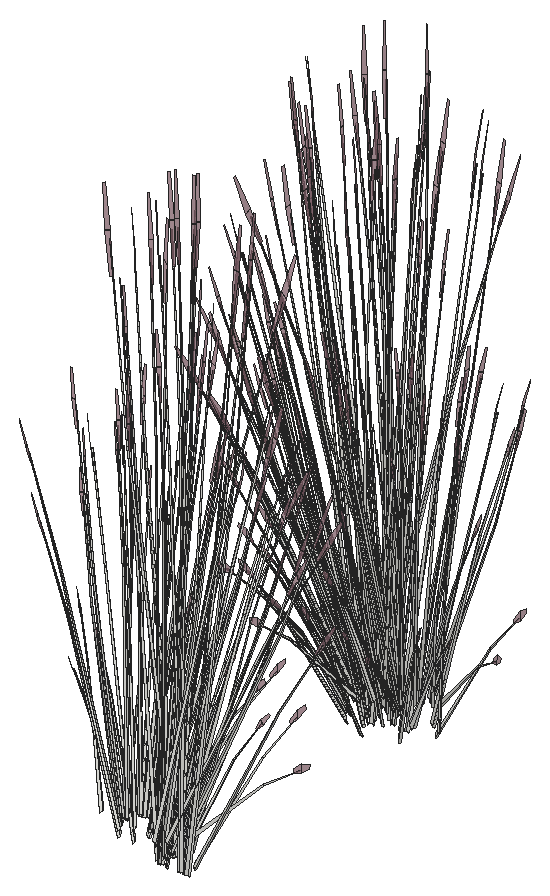
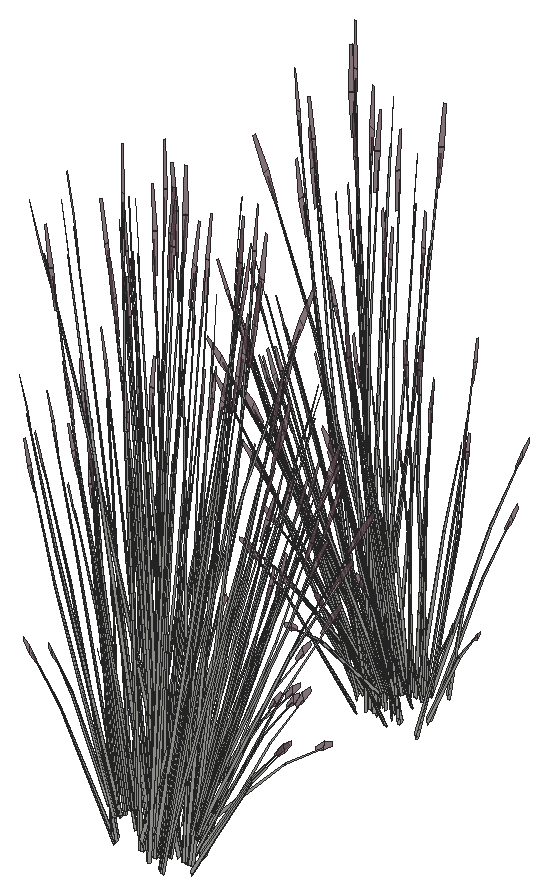
# SketchUp Ruby script. Lengths in inches.
U = 1.inch
M = Sketchup.active_model
def pt(a) = Geom::Point3d.new(a.map { |v| v * U })
def face(e, loops, mat)
  f = e.add_face(loops[0].map { |a| pt(a) })
  loops[1..].each { |l| e.add_face(l.map { |a| pt(a) }).erase! }
  f.material = f.back_material = mat if mat
  f
end
# faces: each face lists its corners as indices into pts; further lists are holes
def faces(e, pts, list, mat = nil) = list.each { |f| face(e, (f[0].is_a?(Array) ? f : [f]).map { |l| l.map { |i| pts[i] } }, mat) }
# xy, xz, yz: faces in a plane at the given z, y or x. An outline is a flat list of corners, or four numbers for a rectangle; further outlines are holes
def ring(l) = l.size == 4 ? [[l[0], l[1]], [l[2], l[1]], [l[2], l[3]], [l[0], l[3]]] : l.each_slice(2).to_a
def flat(e, list, mat, &to3) = list.each { |f| face(e, (f[0].is_a?(Array) ? f : [f]).map { |l| ring(l).map { |u, v| to3.(u, v) } }, mat) }
def xy(e, z, list, mat = nil) = flat(e, list, mat) { |x, y| [x, y, z] }
def xz(e, y, list, mat = nil) = flat(e, list, mat) { |x, z| [x, y, z] }
def yz(e, x, list, mat = nil) = flat(e, list, mat) { |y, z| [x, y, z] }
def lines(e, pts, list) = list.each { |a, b| e.add_line(pt(pts[a]), pt(pts[b])) }
# prism: a flat outline (further loops are holes) pulled along v
def prism(e, loops, v, mat = nil)
  f = face(e, loops, mat); d = Geom::Vector3d.new(v.map { |x| x * U })
  f.pushpull(f.normal.samedirection?(d) ? d.length : -d.length)
end
def box(e, o, s, mat = nil) = prism(e, [[o, [o[0] + s[0], o[1], o[2]], [o[0] + s[0], o[1] + s[1], o[2]], [o[0], o[1] + s[1], o[2]]]], [0, 0, s[2]], mat)
def at(x, y, z, deg = 0) = Geom::Transformation.translation(pt([x, y, z])) * Geom::Transformation.rotation(ORIGIN, Z_AXIS, deg.degrees)
def axes(o, x, y, z) = Geom::Transformation.new([*x, 0, *y, 0, *z, 0, *pt(o).to_a, 1])
def part(name) = M.definitions.add(name)
# library, detail: a bought-in or finely detailed component or shape, given as its bounding box
def library(name, o, s) = part(name).tap { |d| box(d.entities, o, s) }
def detail(e, o, s) = box(e.add_group.entities, o, s)
def put(e, d, t, mat = nil) = e.add_instance(d, t).tap { |i| i.material = mat if mat }
def group(e, t, mat = nil) = e.add_group.tap { |g| g.transformation = t; g.material = mat if mat }.entities
root = M.entities
M.materials.add("LightPink_Translucent").color = [144, 107, 117]
M.materials["LightPink_Translucent"].alpha = 0.75
c1 = part("blade")
p = [[2.15,0.21,22],[0,0.17,0],[0.09,0.45,0],[2.18,0.31,22],[2.29,0.31,22],[0.38,0.45,0],
  [2.48,0.24,33],[2.49,0.24,33],[2.48,0.22,33]]
faces(c1.entities,p,[[0,1,2,3],[4,5,2,3],[6,3,4,7],[8,0,3,6]])
c2 = part("seeds")
p = [[0.3,-0.1,1.38],[-0.01,-0.03,1.59],[-0.01,-0.03,0.03],[0.14,-0.07,-0.07],[0.29,-0.03,3],[0.15,0.01,3.11]]
faces(c2.entities,p,[[0,1,2,3],[1,0,4,5]],"LightPink_Translucent")
c3 = part("blade with seeds")
put(c3.entities,c1,at(0,0,0))
put(c3.entities,c2,axes([2.4,0.25,30.99],[1.5799,-0.05474,1.17369],[-0.12525,1.92788,0.29478],[-0.07173,-0.02425,1.56792]))
put(root,c3,axes([360.53,227.94,49.94],[-0.13408,-0.12117,1.07251],[0.17446,-0.40083,-0.23066],[0.27128,0.0543,0.45856]))
put(root,c3,axes([358.14,228.38,49.65],[0.56127,0.22118,0],[-0.27012,0.45959,0],[0,0,1.31215]))
put(root,c3,axes([359.76,228.125,51.54],[0.11943,-0.00833,1.31208],[0.32759,-0.38275,-0.2075],[0.21244,0.05052,0.10523]))
put(root,c3,axes([358.36,228.87,49.64],[-0.34375,-0.4954,-0.03857],[0.58235,-0.27531,0.38706],[-0.1435,0.04717,1.22723]))
put(root,c3,axes([358.24,227.67,49.96],[0.41131,0.296,0.1086],[-0.34309,0.33395,-0.3101],[-0.0955,0.04515,0.95058]))
put(root,c3,axes([354.99,227.75,51.55],[-0.13808,-0.45342,0.36002],[0.54163,-0.07869,0.29685],[-0.15963,0.10664,0.74497]))
put(root,c3,axes([354.88,227.66,51.55],[-0.3822,-0.20719,0.04823],[0.22252,-0.29505,0.37966],[-0.12254,0.09539,0.57892]))
put(root,c3,axes([355.06,227.12,50.91],[0.19317,-0.10421,1.28532],[0.16263,0.48153,0.10393],[-0.30326,0.10883,0.54946]))
put(root,c3,axes([359.3,228.1875,51.74],[0.55654,0.01186,-0.53284],[-0.03738,0.49951,0.0643],[0.23578,0.05271,0.75375]))
put(root,c3,axes([358.67,228.59,49.86],[0.52105,-0.24633,0.37238],[0.31144,0.44171,0],[-0.11867,0.0561,1.18128]))
put(root,c3,axes([357.93,228.2,49.72],[0.24206,0.56598,-0.04509],[-0.69162,0.19832,0],[0.00845,0.01976,1.2913]))
put(root,c3,axes([358.2,228.81,49.52],[-0.51941,-0.1219,-0.23233],[0.13078,-0.42928,0.23233],[-0.10471,0.0495,1.0423]))
put(root,c3,axes([354.45,227.9375,49.94],[0.19348,0.04044,1.07251],[0.1247,0.41309,-0.23066],[-0.26282,0.07733,0.45856]))
put(root,c3,axes([355.32,227.6,51.79],[0.48462,-0.07041,0.2656],[0.12797,0.4025,-0.3429],[-0.13888,0.10811,0.65611]))
put(root,c3,axes([360.21,227.17,49.78],[0.69617,0,0],[0,0.55062,-0.38706],[0,0.12541,1.22783]))
put(root,c3,axes([353.46,227.42,51.53],[0.07105,0.01321,1.33037],[0.2198,0.43529,-0.12571],[-0.14545,0.11425,0.23543]))
put(root,c3,axes([359.93,227.46,49.65],[-0.69582,-0.00394,-0.03732],[0,-0.55062,0.37457],[-0.02187,0.12535,1.18764]))
put(root,c3,axes([358.43,226.98,50],[0.62699,0.23507,-0.21822],[-0.3019,0.49615,-0.37502],[0.0197,0.12182,1.19781]))
put(root,c3,axes([354.05,228.8,50.07],[0.23202,-0.22328,0.86145],[0.09155,0.35348,0.63294],[-0.16768,0.06329,0.18974]))
put(root,c3,axes([359.64,228.39,51.39],[0.31678,0.30846,-0.2656],[-0.36171,0.29199,0.3429],[0.18378,0.04443,0.65611]))
put(root,c3,axes([359.79,227.54,49.52],[-0.38863,0.30738,-0.23233],[-0.38863,-0.30738,0.23233],[0,0.09901,1.0423]))
put(root,c3,axes([358.11,227.57,50],[0.06488,0.56215,-0.21822],[-0.6757,0.03399,-0.37502],[-0.11898,0.07488,1.19781]))
put(root,c3,axes([359.47,228.51,51.55],[-0.02803,0.37463,0.04823],[-0.42332,-0.01027,0.37966],[0.16216,0.0392,0.57892]))
put(root,c3,axes([358.36,227.35,49.66],[-0.27012,0.44393,-0.33554],[-0.56127,-0.21365,0.16149],[0,0.10233,1.07733]))
put(root,c3,axes([354.93,227.84,51.39],[-0.48462,0.07041,-0.2656],[-0.12797,-0.4025,0.3429],[-0.13888,0.10811,0.65611]))
put(root,c3,axes([359.51,228.39,51.55],[-0.41051,0.32462,0.36002],[-0.35404,-0.34474,0.29685],[0.1926,0.05988,0.74497]))
put(root,c3,axes([354.22,228.74,52.23],[0.49129,0.13151,-0.04866],[-0.15113,0.40475,-0.22062],[-0.08035,0.06145,0.72768]))
put(root,c3,axes([357.71,227.99,49.54],[-0.375,0.3703,-0.46765],[-0.46584,-0.33578,-0.12274],[-0.15027,0.09237,1.03225]))
put(root,c3,axes([358.21,228.77,51.79],[-0.08599,-0.39682,0.2656],[0.49155,-0.10478,-0.3429],[0.13203,0.11372,0.65611]))
put(root,c3,axes([358.375,228.62,49.75],[0.697,0.16013,0.23067],[-0.17437,0.57237,-0.27369],[-0.11536,0.07164,1.23664]))
put(root,c3,axes([358.32,229,49.51],[-0.52105,0.24633,-0.37238],[-0.31144,-0.44171,0],[-0.11867,0.0561,1.18128]))
put(root,c3,axes([360.06,227.55,49.51],[0,0.49266,-0.37238],[-0.62289,0,0],[0,0.11221,1.18128]))
put(root,c3,axes([358.5,227.6,50.91],[-0.2068,-0.08488,1.28532],[0.42797,-0.35609,0.10393],[0.26673,0.16064,0.54946]))
put(root,c3,axes([358.54,226.48,51.36],[-0.48108,-0.25598,1.03712],[0.50798,-0.39855,0.44749],[0.15521,0.24018,1.00248]))
put(root,c3,axes([355.07,227.5625,51.78],[0.515,0.27165,-0.0912],[-0.2967,0.3934,-0.50621],[-0.1455,0.13675,0.76918]))
put(root,c3,axes([359.26,228.57,50.07],[-0.31347,-0.14166,0.86145],[0.40476,-0.14393,0.63294],[0.10917,0.12192,0.18974]))
put(root,c3,axes([358.16,228.97,51.78],[0.33176,-0.4217,-0.0912],[0.48044,0.24295,-0.50621],[0.16701,0.11914,0.76918]))
put(root,c3,axes([355.76,227.44,50.91],[0.13906,-0.15138,1.28532],[0.35111,0.40859,0.10393],[-0.24082,0.18608,0.54946]))
put(root,c3,axes([355.33,227.89,51.51],[0.14302,0.44985,-0.38324],[-0.54163,0.07869,-0.29685],[-0.15522,0.12083,0.7333]))
put(root,c3,axes([355.98,228.4,51.79],[0.3767,-0.25939,0.2656],[0.3566,0.29618,-0.3429],[-0.05426,0.15048,0.65611]))
put(root,c3,axes([358.8,228.93,49.78],[0.34808,0.49367,0],[-0.58235,0.27531,-0.38706],[-0.13264,0.0627,1.22783]))
put(root,c3,axes([357.73,229.32,51.53],[0.00165,-0.05965,1.33037],[0.47711,-0.26315,-0.12571],[0.16572,0.09393,0.23543]))
put(root,c3,axes([359.35,229.09,49.12],[0.04056,-0.07113,1.32257],[0.51066,-0.20948,-0.20205],[0.15482,0.10842,0.22528]))
put(root,c3,axes([358.5,226.97,50.13],[-0.01521,-0.46386,1.05954],[0.68831,0.12024,0.44862],[-0.1628,0.25382,1.00012]))
put(root,c3,axes([358.68,227.48,49.57],[0.20414,0.45107,-0.51909],[-0.58805,0.16245,-0.13624],[0.02256,0.15274,1.1458]))
put(root,c3,axes([355.63,228.64,51.55],[-0.45752,-0.02296,0.04823],[0.01254,-0.34663,0.37966],[-0.04787,0.13278,0.57892]))
put(root,c3,axes([354.66,229.03,49.12],[0.07468,0.04922,1.32257],[0.12663,0.45605,-0.20205],[-0.16551,0.09725,0.22528]))
put(root,c3,axes([355.78,228.67,51.55],[-0.39645,-0.33614,0.36002],[0.42102,-0.2899,0.29685],[-0.07313,0.15771,0.74497]))
put(root,c3,axes([358.56,228.76,51.51],[0.54938,-0.11711,-0.38324],[0.0961,0.44351,-0.29685],[0.14756,0.1271,0.7333]))
put(root,c3,axes([357.03,228.83,51.79],[0.16784,-0.37886,0.2656],[0.48968,0.1105,-0.3429],[0.0449,0.15254,0.65611]))
put(root,c3,axes([359.3125,229.21,50],[-0.35702,-0.01545,0.78795],[0.23577,-0.32816,0.43504],[0.14104,0.11659,0.61808]))
put(root,c3,axes([358.29,229.125,51.55],[-0.25304,0.31296,0.04823],[-0.36033,-0.18221,0.37966],[0.11649,0.10034,0.57892]))
put(root,c3,axes([357.69,230.18,52.23],[0.38473,-0.28263,-0.04866],[0.35252,0.30954,-0.22062],[0.02482,0.08771,0.72768]))
put(root,c3,axes([358.39,229.04,51.55],[-0.55374,0.11306,0.36002],[-0.0961,-0.44351,0.29685],[0.13023,0.13071,0.74497]))
put(root,c3,axes([355.66,227.82,50.91],[0.10366,-0.16934,1.28532],[0.43488,0.35044,0.10393],[-0.19618,0.21841,0.54946]))
put(root,c3,axes([358.15,228.42,49.94],[0.00982,-0.16331,1.07251],[0.4695,-0.18242,-0.23066],[0.14493,0.19547,0.45856]))
put(root,c3,axes([356.88,229.17,51.55],[-0.41024,0.16744,0.04823],[-0.2008,-0.30532,0.37966],[0.03962,0.13459,0.57892]))
put(root,c3,axes([355.78,228.77,51.39],[-0.3767,0.25939,-0.2656],[-0.3566,-0.29618,0.3429],[-0.05426,0.15048,0.65611]))
put(root,c3,axes([354.48,228.69,51.54],[-0.01384,0.09749,1.31208],[0.39274,0.33916,-0.2075],[-0.10282,0.16039,0.10523]))
put(root,c3,axes([355.74,228.47,52.05],[0.61188,0.02441,-0.10123],[-0.01672,0.46217,-0.56189],[-0.0425,0.178,0.85379]))
put(root,c3,axes([356.87,228.99,51.78],[0.54481,-0.22937,-0.0912],[0.26773,0.4071,-0.50621],[0.07188,0.17155,0.76918]))
put(root,c3,axes([357.03,229.14,51.8],[-0.54859,-0.1288,0.39962],[0.18759,-0.42344,0.32951],[0.03297,0.16652,0.82692]))
put(root,c3,axes([356.02,229.78,50.07],[-0.01441,-0.29294,0.86145],[0.36003,0.20894,0.63294],[-0.07081,0.13963,0.18974]))
put(root,c3,axes([356.97,229.08,49.12],[0.0901,-0.02681,1.32257],[0.54199,0.14755,-0.20205],[0.01585,0.1663,0.22528]))
put(root,c3,axes([356.15,228.65,51.75],[0.39855,0.33102,-0.4254],[-0.42102,0.2899,-0.32951],[-0.06064,0.16819,0.81396]))
put(root,c3,axes([355.72,229.15,50.12],[0.50577,-0.08724,0.04881],[0.11627,0.35148,-0.64728],[-0.03206,0.17792,0.5802]))
put(root,c3,axes([357.34,228.97,51.51],[0.54728,0.1235,-0.38324],[-0.18759,0.42344,-0.29685],[0.05018,0.17048,0.7333]))
put(root,c3,axes([357.65,228.1,50.91],[-0.12726,-0.15818,1.28532],[0.58807,-0.13317,0.10393],[0.13291,0.24832,0.54946]))
put(root,c3,axes([357.09,229.23,51.39],[-0.16784,0.37886,-0.2656],[-0.48968,-0.1105,0.3429],[0.0449,0.15254,0.65611]))
put(root,c3,axes([356.03,228.5,52],[-0.01449,0.45571,-0.59145],[-0.61002,-0.03061,0.07138],[-0.06438,0.19306,0.83667]))
put(root,c3,axes([354.4375,229.69,51.53],[0.06316,-0.02974,1.33037],[0.52204,0.19785,-0.12571],[-0.01227,0.16473,0.23543]))
put(root,c3,axes([356.61,228.17,50.91],[-0.01363,-0.18909,1.28532],[0.5906,0.12544,0.10393],[-0.03653,0.26947,0.54946]))
put(root,c3,axes([357.14,228.89,51.74],[0.26572,0.40059,-0.53284],[-0.54698,0.22325,0.0643],[0.06214,0.19355,0.75375]))
put(root,c3,axes([355.6,229.52,49.94],[0.17569,-0.07772,1.07251],[0.43377,0.23434,-0.23066],[-0.12911,0.20277,0.45856]))
put(root,c3,axes([356.74,229.9,51.54],[0.07057,0.07933,1.31208],[0.56952,0.03117,-0.2075],[0.05727,0.17496,0.10523]))
put(root,c3,axes([355.83,229.14,50.52],[0.01223,-0.25433,1.15759],[0.55017,0.13434,0.15997],[-0.04767,0.27105,0.54661]))
put(root,c3,axes([356.25,248.83,50.91],[0.12726,0.15818,1.28532],[-0.58807,0.13317,0.10393],[-0.13291,-0.24832,0.54946]))
put(root,c3,axes([357.22,247.78,51.54],[-0.08515,-0.06907,1.31208],[-0.56828,0.04379,-0.2075],[-0.0907,-0.16522,0.10523]))
put(root,c3,axes([358.54,248.6,49.94],[-0.15825,0.09972,1.07251],[-0.47395,-0.17454,-0.23066],[0.08785,-0.21706,0.45856]))
put(root,c3,axes([357.82,248.94,51.74],[-0.26572,-0.40059,-0.53284],[0.54698,-0.22325,0.0643],[-0.06214,-0.19355,0.75375]))
put(root,c3,axes([356.09,248.41,49.94],[-0.03371,0.16116,1.07251],[-0.49286,0.13491,-0.23066],[-0.11521,-0.20831,0.45856]))
put(root,c3,axes([357.36,248.06,49.12],[-0.09338,0.01775,1.32257],[-0.51641,-0.1998,-0.20205],[0.00867,-0.16666,0.22528]))
put(root,c3,axes([358.92,249.34,51.74],[0.01449,-0.45571,-0.53284],[0.61002,0.03061,0.0643],[0.06438,-0.19306,0.75375]))
put(root,c3,axes([359.77,248.625,51.54],[-0.00537,-0.09805,1.31208],[-0.45391,-0.28338,-0.2075],[0.07018,-0.17178,0.10523]))
put(root,c3,axes([357.87,248.6,51.39],[0.16784,-0.37886,-0.2656],[0.48968,0.1105,0.3429],[-0.0449,-0.15254,0.65611]))
put(root,c3,axes([358.24,249.1,50.91],[-0.10366,0.16934,1.28532],[-0.43488,-0.35044,0.10393],[0.19618,-0.21841,0.54946]))
put(root,c3,axes([359.65,248.27,51.53],[-0.05654,0.03763,1.33037],[-0.55396,-0.12696,-0.12571],[-0.02005,-0.16422,0.23543]))
put(root,c3,axes([357.62,248.86,51.51],[-0.54728,-0.1235,-0.38324],[0.18759,-0.42344,-0.29685],[-0.05018,-0.17048,0.7333]))
put(root,c3,axes([357.95,247.8,50.07],[0.07142,0.28728,0.86145],[-0.3962,-0.15911,0.63294],[0.04263,-0.1471,0.18974]))
put(root,c3,axes([358.8,249.18,51.51],[-0.39855,-0.33102,-0.38324],[0.42102,-0.2899,-0.29685],[0.06064,-0.16819,0.7333]))
put(root,c3,axes([356.64,247.55,51.53],[-0.01039,0.05905,1.33037],[-0.51226,0.21431,-0.12571],[-0.15074,-0.10955,0.23543]))
put(root,c3,axes([356.52,248.6,51.82],[0.62019,-0.12663,0.40322],[0.10763,0.49673,0.33247],[-0.14586,-0.1464,0.83437]))
put(root,c3,axes([357.93,248.69,51.55],[0.54859,0.1288,0.36002],[-0.18759,0.42344,0.29685],[-0.03297,-0.16652,0.74497]))
put(root,c3,axes([358.08,248.84,51.78],[-0.54481,0.22937,-0.0912],[-0.26773,-0.4071,-0.50621],[-0.07188,-0.17155,0.76918]))
put(root,c3,axes([359.22,249.36,51.78],[-0.61188,-0.02441,-0.0912],[0.01672,-0.46217,-0.50621],[0.0425,-0.178,0.76918]))
put(root,c3,axes([359.17,249.0625,51.39],[0.3767,-0.25939,-0.2656],[0.3566,0.29618,0.3429],[0.05426,-0.15048,0.65611]))
put(root,c3,axes([355.92,248.15,50.07],[0.29042,0.17147,0.86145],[-0.42295,0.10307,0.63294],[-0.0905,-0.13178,0.18974]))
put(root,c3,axes([358.07,248.66,51.55],[0.41024,-0.16744,0.04823],[0.2008,0.30532,0.37966],[-0.03962,-0.13459,0.57892]))
put(root,c3,axes([356.62,249.06,51.74],[-0.47473,-0.23813,-0.53284],[0.33738,-0.41728,0.0643],[-0.172,-0.14218,0.75375]))
put(root,c3,axes([356.45,248.74,51.39],[-0.08599,-0.39682,-0.2656],[0.49155,-0.10478,0.3429],[-0.13203,-0.11372,0.65611]))
put(root,c3,axes([356.67,248.71,51.55],[0.25304,-0.31296,0.04823],[0.36033,0.18221,0.37966],[-0.11649,-0.10034,0.57892]))
put(root,c3,axes([355.6875,248.67,49.12],[-0.05393,0.0649,1.32257],[-0.545,0.13993,-0.20205],[-0.13166,-0.12729,0.22528]))
put(root,c3,axes([356.59,250.45,49.57],[-0.22864,-0.5052,-0.52377],[0.65862,-0.18195,-0.13747],[-0.02527,-0.17107,1.15612]))
put(root,c3,axes([355.4,249.32,50.91],[0.2068,0.08488,1.28532],[-0.42797,0.35609,0.10393],[-0.26673,-0.16064,0.54946]))
put(root,c3,axes([359.64,248.9,49.12],[-0.08333,-0.03881,1.32257],[-0.21404,-0.4336,-0.20205],[0.14439,-0.11767,0.22528]))
put(root,c3,axes([357.92,249,51.79],[-0.16784,0.37886,0.2656],[-0.48968,-0.1105,-0.3429],[-0.0449,-0.15254,0.65611]))
put(root,c3,axes([356.4,249.07,51.51],[-0.54938,0.11711,-0.38324],[-0.0961,-0.44351,-0.29685],[-0.14756,-0.1271,0.7333]))
put(root,c3,axes([359.17,249.16,51.55],[0.39645,0.33614,0.36002],[-0.42102,0.2899,0.29685],[0.07313,-0.15771,0.74497]))
put(root,c3,axes([356.78,248.67,52.07],[-0.37157,0.4723,-0.10215],[-0.5381,-0.2721,-0.56695],[-0.18705,-0.13344,0.86148]))
put(root,c3,axes([359.32,249.19,51.55],[0.45752,0.02296,0.04823],[-0.01254,0.34663,0.37966],[0.04787,-0.13278,0.57892]))
put(root,c3,axes([358.98,249.43,51.79],[-0.3767,0.25939,0.2656],[-0.3566,-0.29618,-0.3429],[0.05426,-0.15048,0.65611]))
put(root,c3,axes([359.64,250.13,51.74],[0.29081,-0.38873,-0.53284],[0.5096,0.27626,0.0643],[0.17364,-0.14084,0.75375]))
put(root,c3,axes([356.5,249,49.78],[-0.34808,-0.49367,0],[0.58235,-0.27531,-0.38706],[0.13264,-0.0627,1.22783]))
put(root,c3,axes([359.625,249.95,51.51],[-0.14302,-0.44985,-0.38324],[0.54163,-0.07869,-0.29685],[0.15522,-0.12083,0.7333]))
put(root,c3,axes([357.26,248.4,49.6],[-0.38473,0.28263,-0.02919],[-0.35252,-0.30954,-0.13237],[-0.02482,-0.08771,0.43661]))
put(root,c3,axes([355.36,248.54,51.54],[-0.11979,-0.00348,1.31208],[-0.38137,0.34775,-0.2075],[-0.20349,-0.07106,0.10523]))
put(root,c3,axes([359.88,250.27,51.78],[-0.515,-0.27165,-0.0912],[0.2967,-0.3934,-0.50621],[0.1455,-0.13675,0.76918]))
put(root,c3,axes([357.75,251.75,50.49],[0.48111,0.19866,1.13446],[-0.47133,0.42798,0.44862],[-0.21112,-0.25366,0.95105]))
put(root,c3,axes([356.75,249.07,51.79],[0.08599,0.39682,0.2656],[-0.49155,0.10478,-0.3429],[-0.13203,-0.11372,0.65611]))
put(root,c3,axes([355.24,250.38,49.51],[0,-0.49266,-0.37238],[0.62289,0,0],[0,-0.11221,1.18128]))
put(root,c3,axes([356.97,248.92,49.51],[0.52105,-0.24633,-0.37238],[0.31144,0.44171,0],[0.11867,-0.0561,1.18128]))
put(root,c3,axes([360.0625,249.77,49.94],[-0.19889,-0.01459,1.07251],[-0.20376,-0.39145,-0.23066],[0.24434,-0.11074,0.45856]))
put(root,c3,axes([355.27,249.32,51.82],[0.45978,-0.36358,0.40322],[0.39653,0.38611,0.33247],[-0.21571,-0.06707,0.83437]))
put(root,c3,axes([361.15,250.15,51.53],[-0.07272,-0.00374,1.33037],[-0.30197,-0.40092,-0.12571],[0.12127,-0.13182,0.23543]))
put(root,c3,axes([357.59,249.93,49.54],[0.375,-0.3703,-0.46765],[0.46584,0.33578,-0.12274],[0.15027,-0.09237,1.03225]))
put(root,c3,axes([360.29,249.05,50.07],[-0.18544,0.25079,0.86145],[-0.15939,-0.33694,0.63294],[0.15316,-0.08443,0.18974]))
put(root,c3,axes([360.03,249.99,51.39],[0.48462,-0.07041,-0.2656],[0.12797,0.4025,0.3429],[0.13888,-0.10811,0.65611]))
put(root,c3,axes([355.48,249.32,51.55],[0.02803,-0.37463,0.04823],[0.42332,0.01027,0.37966],[-0.16216,-0.0392,0.57892]))
put(root,c3,axes([356.93,250.58,49.66],[0.27012,-0.44393,-0.33554],[0.56127,0.21365,0.16149],[0,-0.10233,1.07733]))
put(root,c3,axes([355.32,249.44,51.39],[-0.31678,-0.30846,-0.2656],[0.36171,-0.29199,0.3429],[-0.18378,-0.04443,0.65611]))
put(root,c3,axes([357.18,250.36,50],[-0.06488,-0.56215,-0.21822],[0.6757,-0.03399,-0.37502],[0.11898,-0.07488,1.19781]))
put(root,c3,axes([355.51,250.39,49.52],[0.38863,-0.30738,-0.23233],[0.38863,0.30738,0.23233],[0,-0.09901,1.0423]))
put(root,c3,axes([355.35,248.92,49.6],[-0.1606,0.40228,-0.02919],[-0.4943,-0.12375,-0.13237],[-0.07505,-0.0658,0.43661]))
put(root,c3,axes([359.63,250.23,51.79],[-0.48462,0.07041,0.2656],[-0.12797,-0.4025,-0.3429],[0.13888,-0.10811,0.65611]))
put(root,c3,axes([356.87,250.95,50],[-0.62699,-0.23507,-0.21822],[0.3019,-0.49615,-0.37502],[-0.0197,-0.12182,1.19781]))
put(root,c3,axes([355.08,250.75,49.78],[-0.69617,0,0],[0,-0.55062,-0.38706],[0,-0.12541,1.22783]))
put(root,c3,axes([355.2,249.77,49.94],[0.1087,0.13716,1.07251],[-0.25048,0.37284,-0.23066],[-0.25719,-0.08912,0.45856]))
put(root,c3,axes([357.09,249.11,49.52],[0.51941,0.1219,-0.23233],[-0.13078,0.42928,0.23233],[0.10471,-0.0495,1.0423]))
put(root,c3,axes([355.65,249.65,51.74],[-0.55654,-0.01186,-0.53284],[0.03738,-0.49951,0.0643],[-0.23578,-0.05271,0.75375]))
put(root,c3,axes([360.07,250.17,51.55],[0.3822,0.20719,0.04823],[-0.22252,0.29505,0.37966],[0.12254,-0.09539,0.57892]))
put(root,c3,axes([359.96,250.08,51.55],[0.13808,0.45342,0.36002],[-0.54163,0.07869,0.29685],[0.15963,-0.10664,0.74497]))
put(root,c3,axes([361.42,250.63,51.54],[0.07726,-0.07504,1.31208],[-0.09888,-0.46032,-0.2075],[0.19384,-0.08728,0.10523]))
put(root,c3,axes([355.625,250.61,49.75],[-0.51786,0.4142,0.23067],[-0.51817,-0.40984,-0.27369],[-0.01808,-0.11762,1.23664]))
put(root,c3,axes([354.9,248.83,51.53],[0.04127,0.04917,1.33037],[-0.19898,0.44196,-0.12571],[-0.20151,0.0032,0.23543]))
put(root,c3,axes([357.27,250.8,49.82],[0.6273,0.23878,0.18048],[-0.3019,0.49615,0.37502],[0,-0.11437,1.20407]))
put(root,c3,axes([357.03,251.47,49.83],[0.14756,-0.58378,-0.17572],[0.69966,0.10176,0.38453],[-0.12225,-0.08062,1.1733]))
put(root,c3,axes([355.47,249.75,51.51],[-0.40426,0.32635,-0.38324],[-0.35404,-0.34474,-0.29685],[-0.2054,-0.04965,0.7333]))
put(root,c3,axes([355.77,249.6,51.79],[0.31678,0.30846,0.2656],[-0.36171,0.29199,-0.3429],[-0.18378,-0.04443,0.65611]))
put(root,c3,axes([354.56,250.18,50.07],[0.35544,-0.03525,0.86145],[-0.22547,0.31061,0.63294],[-0.17565,-0.04659,0.18974]))
put(root,c3,axes([357.07,250.47,50.04],[-0.60457,0.03041,0.33554],[-0.05467,-0.50484,-0.16149],[0.10823,-0.05117,1.07733]))
put(root,c3,axes([355.68,249.41,51.78],[-0.02981,0.50103,-0.0912],[-0.56442,-0.01369,-0.50621],[-0.21738,-0.0348,0.76918]))
put(root,c3,axes([355.51,250.84,49.86],[0,0.49266,0.37238],[-0.62289,0,0],[0,-0.11221,1.18128]))
put(root,c3,axes([359.9,251.33,51.78],[-0.28012,-0.44611,-0.0912],[0.49717,-0.21923,-0.50621],[0.20951,-0.05886,0.76918]))
put(root,c3,axes([359.88,250.94,51.51],[0.15083,-0.44814,-0.38324],[0.51712,0.15361,-0.29685],[0.2082,-0.04109,0.7333]))
put(root,c3,axes([359.0625,249.12,49.78],[0.34808,-0.49367,0],[0.58235,0.27531,-0.38706],[0.13264,0.0627,1.22783]))
put(root,c3,axes([354.96,250.1,50.91],[0.23093,-0.01116,1.28532],[-0.15319,0.4836,0.10393],[-0.32909,-0.02991,0.54946]))
put(root,c3,axes([356.98,251.23,49.66],[-0.33445,-0.41351,-0.33554],[0.50659,-0.29119,0.16149],[-0.10823,-0.05117,1.07733]))
put(root,c3,axes([357.05,250.65,49.77],[0.24206,0.5509,0.34316],[-0.69162,0.19157,0.13466],[0.00845,-0.10123,1.19142]))
put(root,c3,axes([360.43,251.07,49.49],[-0.35858,0.05912,1.06187],[-0.05708,-0.47061,0.06078],[0.25115,-0.07123,0.60425]))
put(root,c3,axes([361.08,250.65,49.7],[-0.34516,-0.31503,-0.04866],[0.37803,-0.28865,-0.22062],[0.10711,-0.02032,0.72768]))
put(root,c3,axes([356.92,251.08,50.04],[-0.27012,0.44393,0.33554],[-0.56127,-0.21365,-0.16149],[0,-0.10233,1.07733]))
put(root,c3,axes([357.92,250.7,49.65],[0,-0.57005,0],[0.69617,0,0],[0,0,1.34592]))
put(root,c3,axes([358.76,249.38,49.86],[-0.52105,-0.24633,0.37238],[0.31144,-0.44171,0],[0.11867,0.0561,1.18128]))
put(root,c3,axes([359.78,251.11,51.74],[0.48922,-0.21758,-0.53284],[0.27264,0.44789,0.0643],[0.23638,-0.05088,0.75375]))
put(root,c3,axes([356.68,251.39,49.54],[-0.57914,-0.08077,-0.46765],[0.12221,-0.49823,-0.12274],[-0.17283,-0.06037,1.03225]))
put(root,c3,axes([357.59,250.34,49.77],[-0.46162,0.4471,0.34316],[-0.54842,-0.39467,0.13466],[0.11129,-0.04462,1.19142]))
put(root,c3,axes([358.09,251.14,49.72],[-0.51786,-0.42404,-0.04598],[0.51817,-0.4243,0],[-0.01808,-0.01481,1.31678]))
put(root,c3,axes([356.79,249.6,49.86],[-0.16083,0.48962,0.13232],[-0.58854,-0.13856,0.26315],[0.10167,-0.00238,1.20305]))
put(root,c3,axes([359.71,251.19,51.79],[-0.46269,-0.13744,0.2656],[0.13495,-0.40096,-0.3429],[0.18628,-0.03677,0.65611]))
put(root,c3,axes([354.86,250.46,51.55],[0.15729,-0.44921,0.36002],[0.51712,0.15361,0.29685],[-0.20336,0.027,0.74497]))
put(root,c3,axes([356.54,250,49.2],[-0.548,0.19724,0.96696],[-0.17442,-0.56594,0.37572],[0.3365,0.00941,1.09981]))
put(root,c3,axes([358.01,250.14,49.96],[0.1074,-0.43968,0.1086],[0.52474,0.07632,-0.3101],[0.0955,0.04515,0.95058]))
put(root,c3,axes([354.83,250.34,51.55],[-0.20448,-0.33592,0.04823],[0.37288,-0.16442,0.37966],[-0.16437,0.03244,0.57892]))
put(root,c3,axes([357.11,251.1875,49.77],[0.70367,0.1038,0.34316],[-0.1432,0.58624,0.13466],[-0.10283,-0.05661,1.19142]))
put(root,c3,axes([360.82,250.76,49.12],[-0.0291,-0.0748,1.32257],[0.20181,-0.43752,-0.20205],[0.20357,-0.00629,0.22528]))
put(root,c3,axes([354.81,250.6875,49.12],[0.01412,0.07764,1.32257],[-0.28464,0.40547,-0.20205],[-0.20218,-0.02044,0.22528]))
put(root,c3,axes([357.79,250.26,50.04],[-0.33445,-0.41351,0.33554],[0.50659,-0.29119,-0.16149],[0.10823,0.05117,1.07733]))
put(root,c3,axes([356.0625,252.15,49.52],[-0.13078,-0.42928,-0.23233],[0.51941,-0.1219,0.23233],[-0.10471,-0.0495,1.0423]))
put(root,c3,axes([356.73,252.125,49.86],[0.59825,-0.13076,0.13232],[0.14773,0.48663,0.26315],[-0.05336,-0.0709,1.20305]))
put(root,c3,axes([357.96,250.29,50],[0.56211,-0.32708,-0.21822],[0.3738,0.46216,-0.37502],[0.13869,0.04694,1.19781]))
put(root,c3,axes([360.2,251.15,51.39],[0.46269,0.13744,-0.2656],[-0.13495,0.40096,0.3429],[0.18628,-0.03677,0.65611]))
put(root,c3,axes([355.92,252.33,49.51],[-0.52105,-0.24633,-0.37238],[0.31144,-0.44171,0],[-0.11867,-0.0561,1.18128]))
put(root,c3,axes([359.38,249.42,49.51],[0.52105,0.24633,-0.37238],[-0.31144,0.44171,0],[0.11867,0.0561,1.18128]))
put(root,c3,axes([354.76,250.51,51.39],[-0.46269,-0.13744,-0.2656],[0.13495,-0.40096,0.3429],[-0.18628,0.03677,0.65611]))
put(root,c3,axes([358.39,250.82,49.65],[0.62289,0,0],[0,0.51004,0],[0,0,1.33805]))
put(root,c3,axes([357.33,251.46,50],[-0.56211,0.32708,-0.21822],[-0.3738,-0.46216,-0.37502],[-0.13869,-0.04694,1.19781]))
put(root,c3,axes([358.57,249.625,49.86],[-0.59825,0.13076,0.13232],[-0.14773,-0.48663,0.26315],[0.05336,0.0709,1.20305]))
